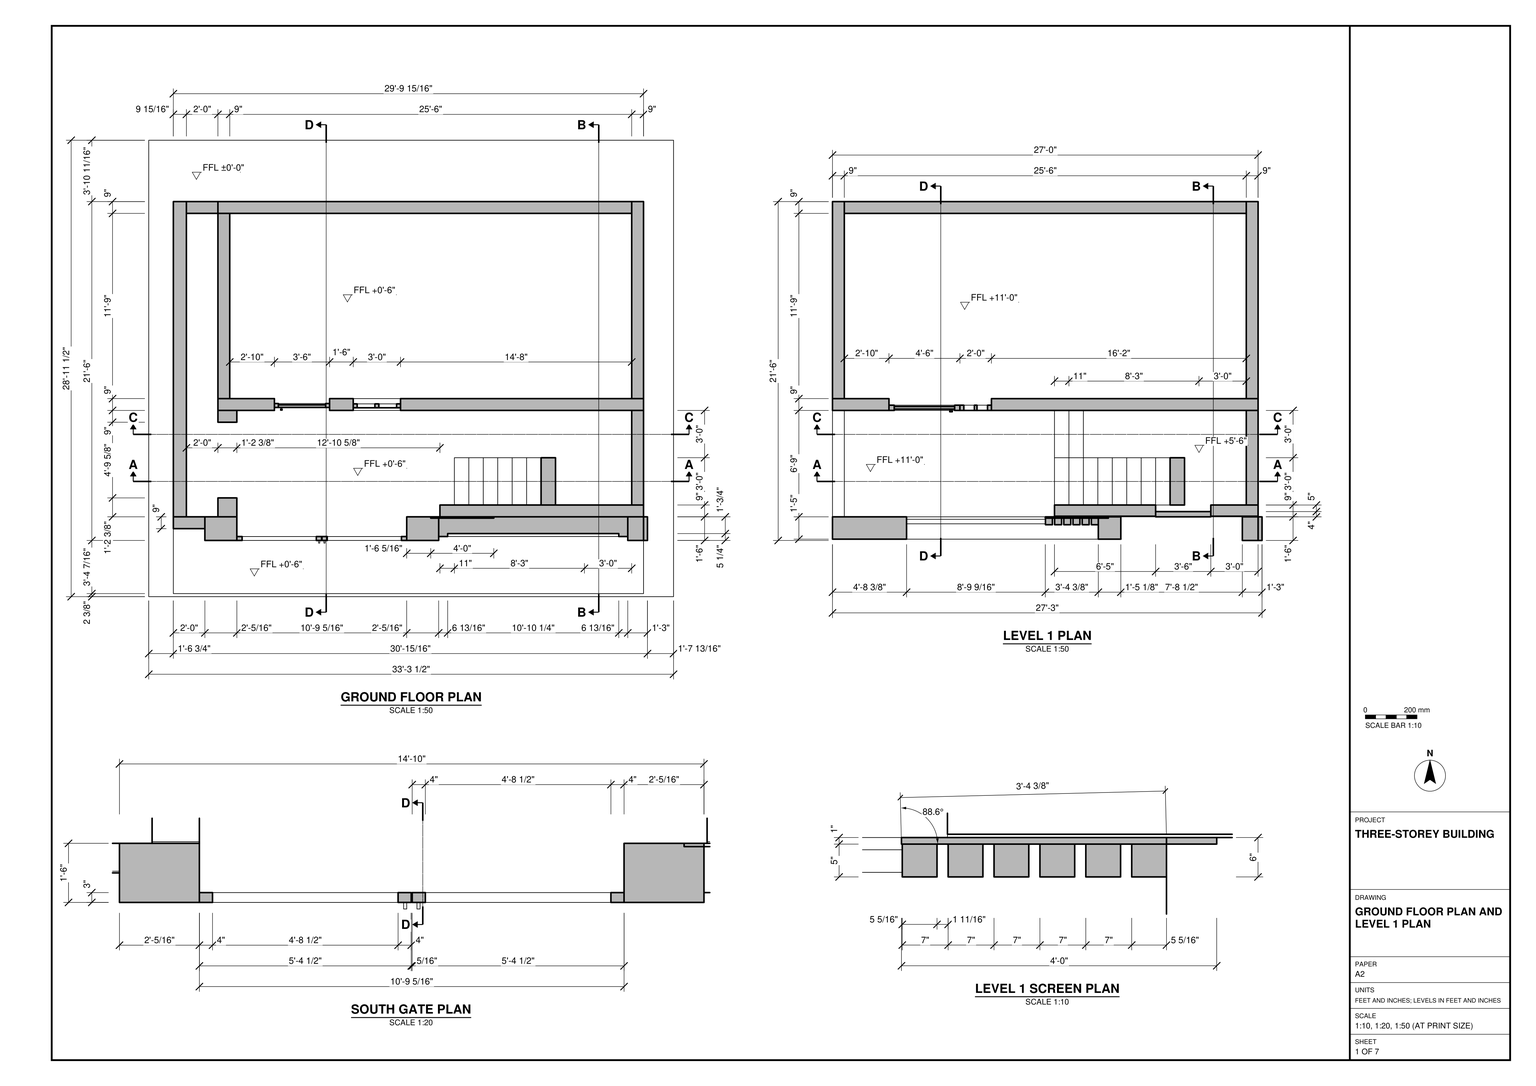
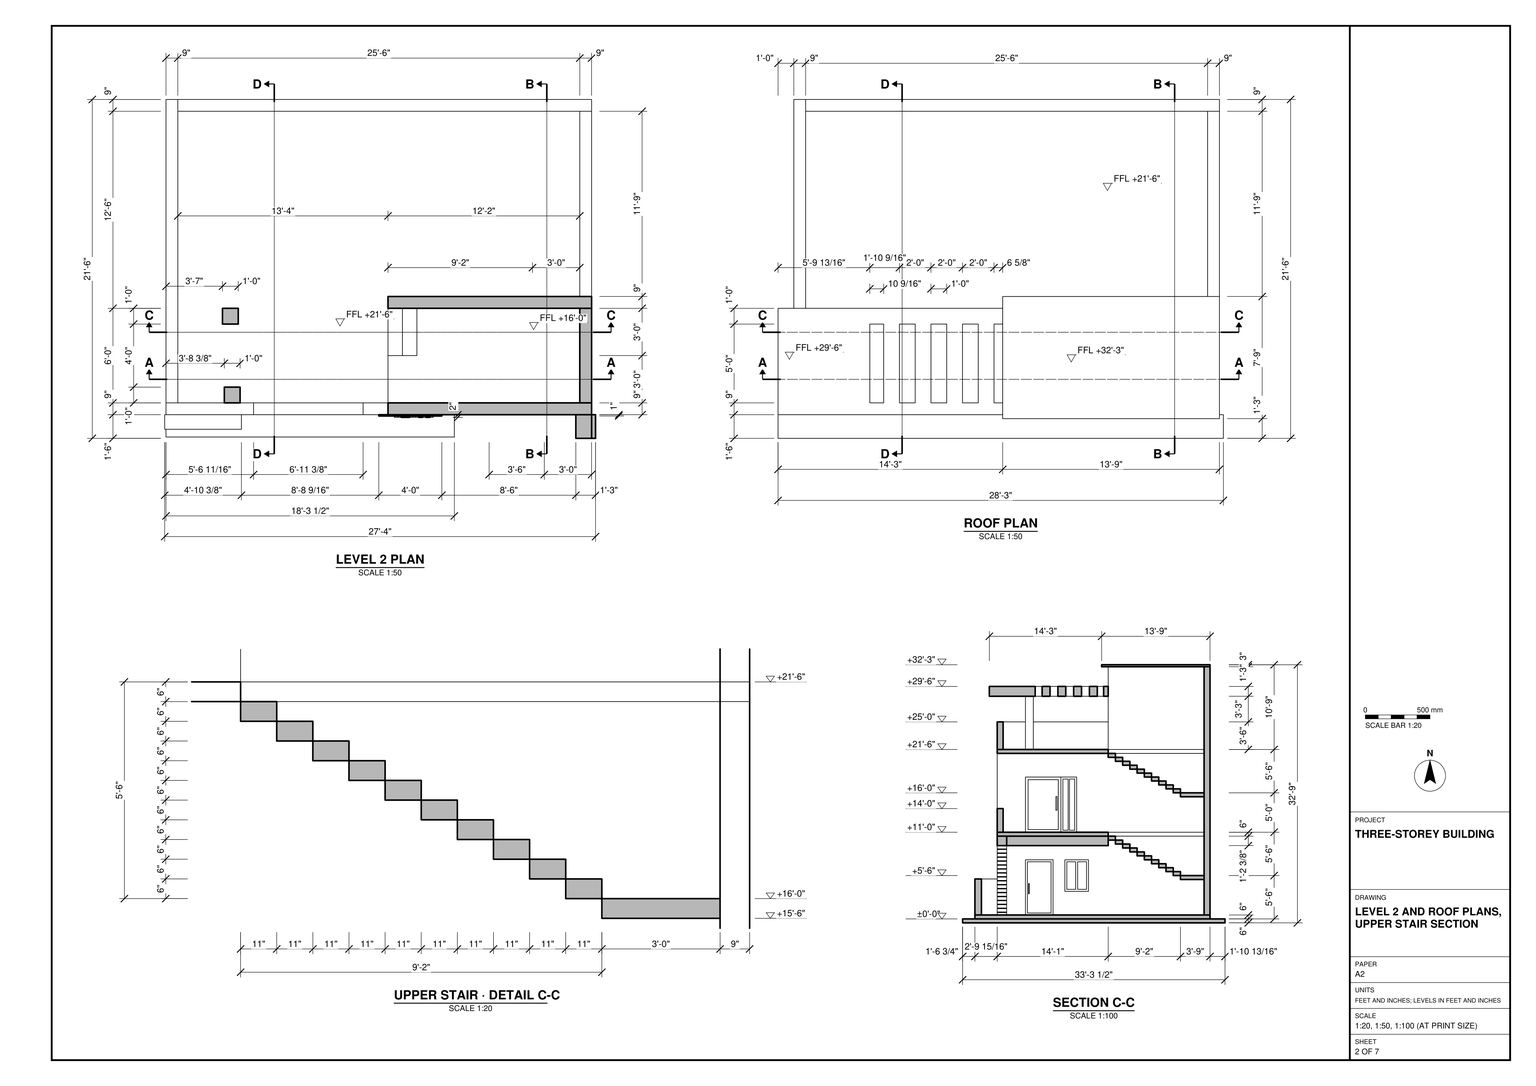
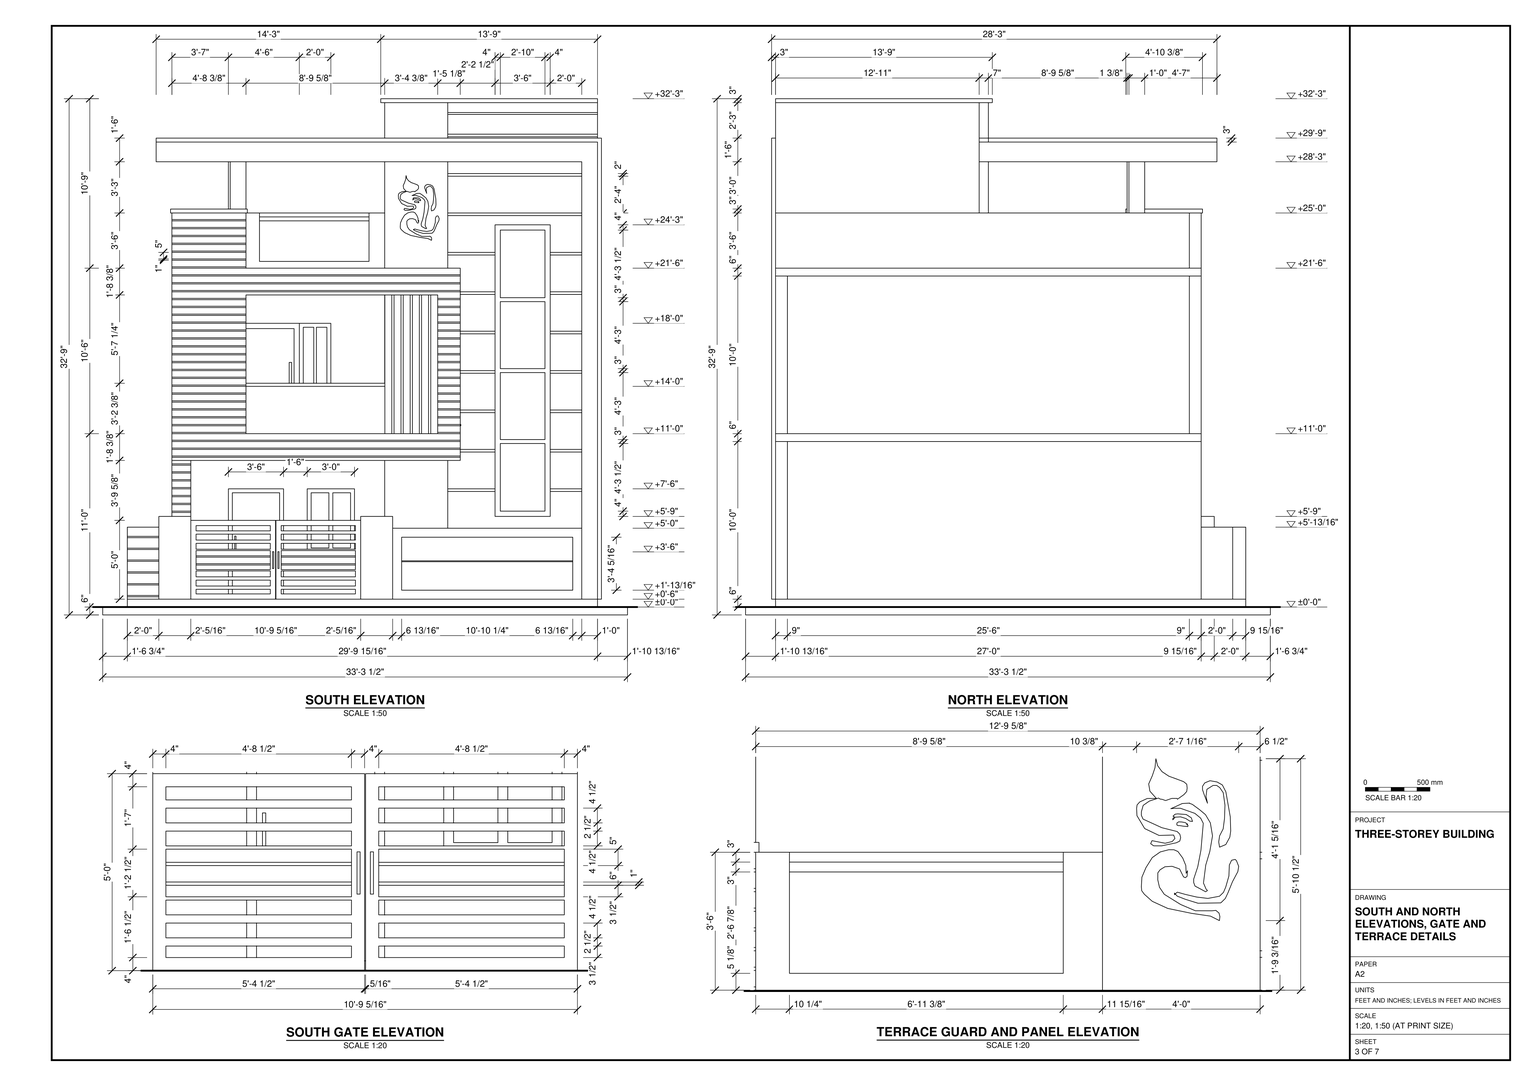
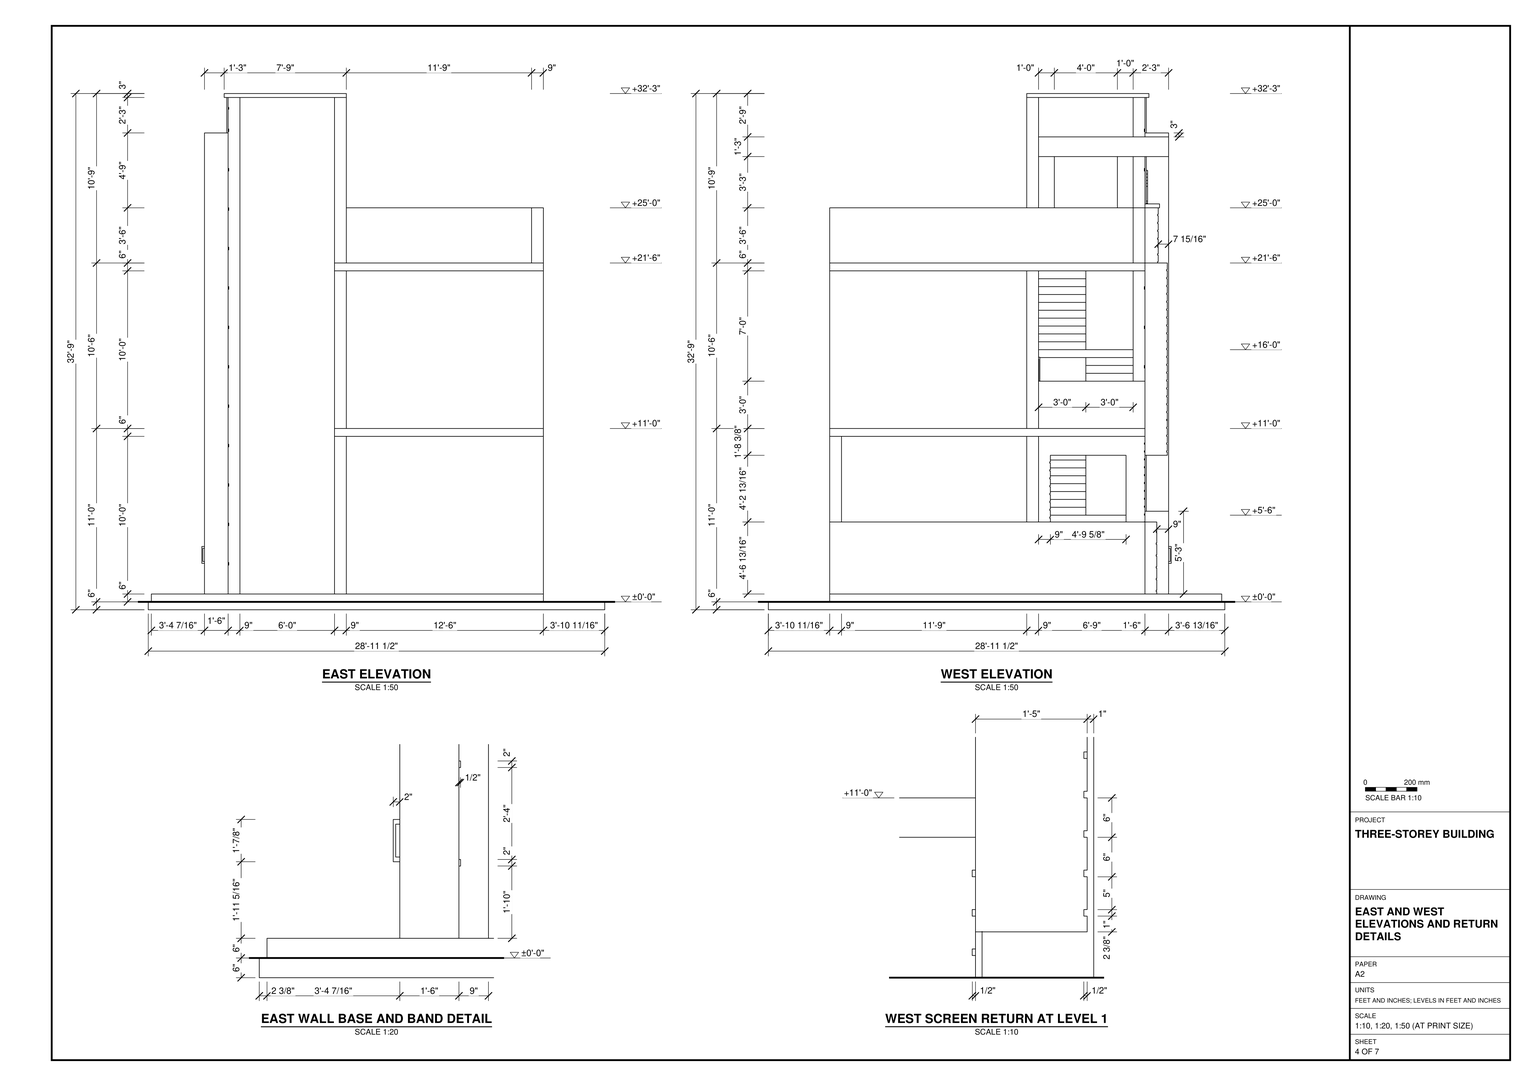
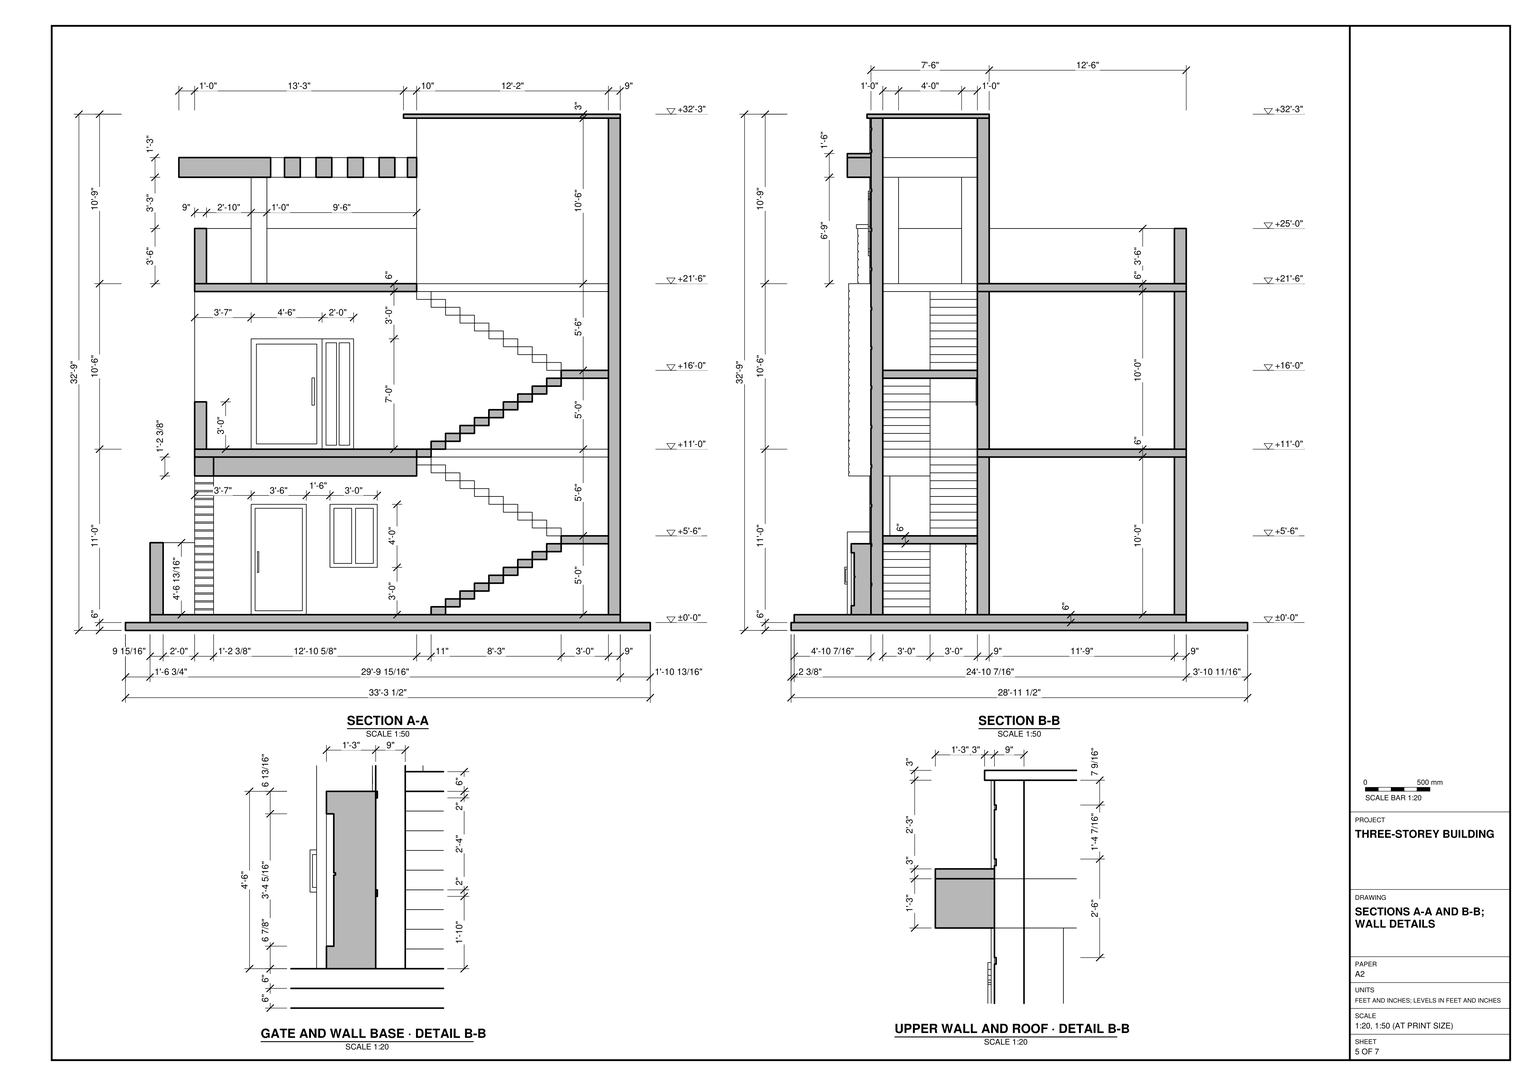
Build the three-storey building in SketchUp from task_files/diagram_01.pdf. Work in feet and inches. Orient the gated frontage to the south. The overall extents, including the base, are 33'-3 1/2" east–west, 28'-11 1/2" north–south and 32'-9" high. Use ±0'-0" as the ground datum, with Level 1 at +11'-0" and Level 2 at +21'-6". Distinguish the raised ground floor at +0'-6" from the surrounding base.

Lay out the walls at the thicknesses shown, with the wide enclosed space to the north and the entrance, stairs and landings to the south. Form the floor slabs around the stair opening and use the sections to connect the flights to their landings. Reproduce the doors and windows in the recessed walls as well as the elements in front of them: the double gate between piers, the horizontally banded balcony frame, the vertical screen and the tall divided panel on the right. At Level 2, model the open terrace, its guard and taller patterned panel. Follow the roof plan for the lower canopy with rectangular openings and the higher solid roof over the stair.

Keep walls, slabs and roof elements in separate groups or components, and group each furniture or joinery piece separately. Use components for repeated parts. Any decor or loose items shown may be suitable library components. Save one SketchUp model as output_files/three_storey_building_with_screened_south_facade.skp.

# SketchUp Ruby script. Lengths in inches.
U = 1.inch
M = Sketchup.active_model
def pt(a) = Geom::Point3d.new(a.map { |v| v * U })
def face(e, loops, mat)
  f = e.add_face(loops[0].map { |a| pt(a) })
  loops[1..].each { |l| e.add_face(l.map { |a| pt(a) }).erase! }
  f.material = f.back_material = mat if mat
  f
end
# faces: each face lists its corners as indices into pts; further lists are holes
def faces(e, pts, list, mat = nil) = list.each { |f| face(e, (f[0].is_a?(Array) ? f : [f]).map { |l| l.map { |i| pts[i] } }, mat) }
# xy, xz, yz: faces in a plane at the given z, y or x. An outline is a flat list of corners, or four numbers for a rectangle; further outlines are holes
def ring(l) = l.size == 4 ? [[l[0], l[1]], [l[2], l[1]], [l[2], l[3]], [l[0], l[3]]] : l.each_slice(2).to_a
def flat(e, list, mat, &to3) = list.each { |f| face(e, (f[0].is_a?(Array) ? f : [f]).map { |l| ring(l).map { |u, v| to3.(u, v) } }, mat) }
def xy(e, z, list, mat = nil) = flat(e, list, mat) { |x, y| [x, y, z] }
def xz(e, y, list, mat = nil) = flat(e, list, mat) { |x, z| [x, y, z] }
def yz(e, x, list, mat = nil) = flat(e, list, mat) { |y, z| [x, y, z] }
def lines(e, pts, list) = list.each { |a, b| e.add_line(pt(pts[a]), pt(pts[b])) }
# prism: a flat outline (further loops are holes) pulled along v
def prism(e, loops, v, mat = nil)
  f = face(e, loops, mat); d = Geom::Vector3d.new(v.map { |x| x * U })
  f.pushpull(f.normal.samedirection?(d) ? d.length : -d.length)
end
def box(e, o, s, mat = nil) = prism(e, [[o, [o[0] + s[0], o[1], o[2]], [o[0] + s[0], o[1] + s[1], o[2]], [o[0], o[1] + s[1], o[2]]]], [0, 0, s[2]], mat)
def at(x, y, z, deg = 0) = Geom::Transformation.translation(pt([x, y, z])) * Geom::Transformation.rotation(ORIGIN, Z_AXIS, deg.degrees)
def axes(o, x, y, z) = Geom::Transformation.new([*x, 0, *y, 0, *z, 0, *pt(o).to_a, 1])
def part(name) = M.definitions.add(name)
# library, detail: a bought-in or finely detailed component or shape, given as its bounding box
def library(name, o, s) = part(name).tap { |d| box(d.entities, o, s) }
def detail(e, o, s) = box(e.add_group.entities, o, s)
def put(e, d, t, mat = nil) = e.add_instance(d, t).tap { |i| i.material = mat if mat }
def group(e, t, mat = nil) = e.add_group.tap { |g| g.transformation = t; g.material = mat if mat }.entities
root = M.entities
M.materials.add("[Color M00]").color = [255, 255, 255]
M.materials.add("[Color M06]").color = [86, 86, 86]
M.materials.add("[Color M07]").color = [58, 58, 58]
M.materials.add("[Metal Silver]").color = [234, 233, 238]
M.materials.add("[Translucent Glass Blue]").color = [100, 149, 237]
M.materials["[Translucent Glass Blue]"].alpha = 0.5
M.materials.add("[Wood Bamboo]").color = [155, 92, 37]
M.materials.add("[Wood Cherry Original]").color = [122, 69, 33]
M.materials.add("[Wood Veneer 01]").color = [86, 50, 26]
c1 = part("Group\#13")
box(c1.entities,[0,0,0],[11,36,6])
c2 = part("Group\#4")
box(c2.entities,[0,0,0],[11,36,6])
c3 = part("Group\#44")
box(c3.entities,[0,0,0],[5.29,5,105.6])
c4 = part("Group\#61")
prism(c4.entities,[[[0.94,2,11.44],[0.94,2,12.875],[0.94,0,12.875],[0.94,0,0],[0.94,2,0],[0.94,2,1.43],[0.94,0.75,1.43],[0.94,0.75,11.44]]],[-0.94,0,0])
c5 = library("Group\#70",[0,0,0],[38.38,2,61.86])
xy(root,44.16,[[100.47,142.05,101.47,144.05]])
xy(root,45.48,[[100.47,142.74,101.47,144.05]])
xy(root,58.65,[[100.47,142.74,101.47,144.05]])
xy(root,60.04,[[100.47,142.05,101.47,144.05]])
xz(root,142.05,[[100.47,44.16,101.47,60.04]],"[Metal Silver]")
xz(root,142.74,[[100.47,45.48,101.47,58.65]])
xz(root,144.05,[[100.47,44.16,101.47,45.48],[100.47,58.65,101.47,60.04]])
yz(root,100.47,[[142.05,44.16,142.05,60.04,144.05,60.04,144.05,58.65,142.74,58.65,142.74,45.48,144.05,45.48,144.05,44.16]])
yz(root,101.47,[[142.05,44.16,144.05,44.16,144.05,45.48,142.74,45.48,142.74,58.65,144.05,58.65,144.05,60.04,142.05,60.04]])
p = [[255.01,60.8,138],[214.66,59.8,138],[214.66,60.8,138],[262.66,60.8,264],[214.66,59.8,264],[262.66,59.8,264],
  [220.71,59.8,75],[214.66,59.8,75],[214.66,60.8,75],[220.71,59.8,66],[262.66,59.8,66],[262.66,60.8,66]]
lines(root,p,[[0,1],[1,2],[3,4],[4,5],[6,7],[7,8],[9,6],[9,10],[10,11]])
g1 = group(root,at(73.125,0,0))
box(g1,[-73.125,0,0],[399.5,347.5,6])
g2 = group(root,at(112.66,60.8,6))
box(g2,[-93.9375,-58.4375,0],[357.9375,298.4375,6])
g3 = group(root,at(232.66,60.8,12))
xy(g3,0,[[-11,0,144,9]])
xy(g3,22,[[-11,0,144,0.5]])
xy(g3,24,[[-11,0,144,0.5]])
xy(g3,52,[[-11,0,144,0.5]])
xy(g3,54,[[-11,0,144,0.5]])
xy(g3,63,[[66,0,108,9]])
xy(g3,82,[[-11,0,66,0.5],[108,0,144,0.5]])
xy(g3,84,[[-11,0,66,0.5],[108,0,144,0.5]])
xy(g3,112,[[-11,0,66,0.5],[108,0,144,0.5]])
xy(g3,114,[[-11,0,66,0.5],[108,0,144,0.5]])
xy(g3,142,[[-11,0,66,0.5],[108,0,144,0.5]])
xy(g3,144,[[-11,0,66,0.5],[108,0,144,0.5]])
xy(g3,172,[[-11,0,66,0.5],[108,0,144,0.5]])
xy(g3,174,[[-11,0,66,0.5],[108,0,144,0.5]])
xy(g3,202,[[-11,0,66,0.5],[108,0,144,0.5]])
xy(g3,204,[[-11,0,66,0.5],[108,0,144,0.5]])
xy(g3,232,[[-11,0,66,0.5],[108,0,144,0.5]])
xy(g3,234,[[-11,0,66,0.5],[108,0,144,0.5]])
xy(g3,262,[[-11,0,66,0.5],[108,0,144,0.5]])
xy(g3,264,[[-11,0,66,0.5],[108,0,144,0.5]])
xy(g3,285,[[66,0,108,9]])
xy(g3,292,[[-11,0,144,0.5]])
xy(g3,294,[[-11,0,144,0.5]])
xy(g3,322,[[-11,0,144,0.5]])
xy(g3,324,[[-11,0,144,0.5]])
xy(g3,352,[[-11,0,144,0.5]])
xy(g3,354,[[-11,0,144,0.5]])
xy(g3,369.03,[[30,0,144,0.5]])
xy(g3,370.46,[[30,0,144,0.5]])
xy(g3,378,[[-11,0,144,9]])
xz(g3,0,[[-11,0,144,22],[-11,24,144,52],[-11,54,144,54,144,82,108,82,108,63,66,63,66,82,-11,82],[-11,84,66,112],[108,84,144,112],
  [-11,114,66,142],[108,114,144,142],[-11,144,66,172],[108,144,144,172],[-11,174,66,202],
  [108,174,144,202],[-11,204,66,232],[108,204,144,232],[-11,234,66,262],[108,234,144,262],
  [-11,264,66,264,66,285,108,285,108,264,144,264,144,292,-11,292],[-11,294,144,322],[-11,324,144,352],[-11,354,144,354,144,369.03,30,369.03,30,370.46,144,370.46,144,378,-11,378]])
xz(g3,0.5,[[-11,22,144,24],[-11,52,144,54],[-11,82,66,84],[108,82,144,84],[-11,112,66,114],
  [108,112,144,114],[-11,142,66,144],[108,142,144,144],[-11,172,66,174],[108,172,144,174],
  [-11,202,66,204],[108,202,144,204],[-11,232,66,234],[108,232,144,234],[-11,262,66,264],
  [108,262,144,264],[-11,292,144,294],[-11,322,144,324],[-11,352,144,354],[30,369.03,144,370.46]])
xz(g3,9,[[[-11,0,144,378],[66,63,108,285]]])
yz(g3,-11,[[0,0,0,22,0.5,22,0.5,24,0,24,0,52,0.5,52,0.5,54,0,54,0,82,0.5,82,0.5,84,0,84,0,112,0.5,112,0.5,114,0,114,0,142,0.5,142,0.5,144,0,144,0,172,0.5,172,0.5,174,0,174,0,202,0.5,202,0.5,204,0,204,0,232,0.5,232,0.5,234,0,234,0,262,0.5,262,0.5,264,0,264,0,292,0.5,292,0.5,294,0,294,0,322,0.5,322,0.5,324,0,324,0,352,0.5,352,0.5,354,0,354,0,378,9,378,9,0]])
yz(g3,30,[[0,369.03,0.5,370.46]])
yz(g3,66,[[0,63,9,63,9,285,0,285,0,264,0.5,264,0.5,262,0,262,0,234,0.5,234,0.5,232,0,232,0,204,0.5,204,0.5,202,0,202,0,174,0.5,174,0.5,172,0,172,0,144,0.5,144,0.5,142,0,142,0,114,0.5,114,0.5,112,0,112,0,84,0.5,84,0.5,82,0,82]])
yz(g3,108,[[0,63,0,82,0.5,82,0.5,84,0,84,0,112,0.5,112,0.5,114,0,114,0,142,0.5,142,0.5,144,0,144,0,172,0.5,172,0.5,174,0,174,0,202,0.5,202,0.5,204,0,204,0,232,0.5,232,0.5,234,0,234,0,262,0.5,262,0.5,264,0,264,0,285,9,285,9,63]])
yz(g3,144,[[0,0,9,0,9,378,0,378,0,370.46,0.5,370.46,0.5,369.03,0,369.03,0,354,0.5,354,0.5,352,0,352,0,324,0.5,324,0.5,322,0,322,0,294,0.5,294,0.5,292,0,292,0,264,0.5,264,0.5,262,0,262,0,234,0.5,234,0.5,232,0,232,0,204,0.5,204,0.5,202,0,202,0,174,0.5,174,0.5,172,0,172,0,144,0.5,144,0.5,142,0,142,0,114,0.5,114,0.5,112,0,112,0,84,0.5,84,0.5,82,0,82,0,54,0.5,54,0.5,52,0,52,0,24,0.5,24,0.5,22,0,22]])
g4 = group(root,at(112.66,141.8,12))
prism(g4,[[[-17,9,0],[-60,9,0],[-60,9,120],[264,9,120],[264,9,0],[25,9,0],[25,9,84],[-17,9,84]],[[79,9,84],[43,9,84],[43,9,36],[79,9,36]]],[0,-9,0])
g5 = group(root,at(367.66,150.8,12))
box(g5,[0,0,0],[9,150,120])
g6 = group(root,at(42.72,291.8,12))
box(g6,[9.9375,0,0],[315,9,120])
g7 = group(root,at(52.66,150.8,12))
box(g7,[0,0,0],[9,141,120])
g8 = group(root,at(52.66,141.8,132))
prism(g8,[[[324,159,0],[324,0,0],[169,0,0],[169,-81,0],[0,-81,0],[0,159,0]]],[0,0,6])
g9 = group(root,at(221.66,69.8,12))
g10 = group(g9,at(11,0,0))
put(g10,c1,at(66,0,36))
put(g10,c1,at(0,0,0))
put(g10,c1,at(55,0,30))
put(g10,c1,at(44,0,24))
put(g10,c1,at(77,0,42))
put(g10,c1,at(88,0,48))
put(g10,c1,at(33,0,18))
put(g10,c1,at(11,0,6))
put(g10,c1,at(22,0,12))
g11 = group(g9,at(110,0,54))
box(g11,[0,0,0],[36,72,6])
put(g9,c1,at(77,72,78,-180))
put(g9,c2,at(11,72,114,-180))
put(g9,c1,at(44,72,96,-180))
put(g9,c1,at(110,72,60,-180))
put(g9,c2,at(22,72,108,-180))
put(g9,c1,at(88,72,72,-180))
put(g9,c1,at(66,72,84,-180))
put(g9,c1,at(99,72,66,-180))
put(g9,c1,at(55,72,90,-180))
put(g9,c1,at(33,72,102,-180))
put(root,c2,at(243.66,141.8,246,-180))
put(root,c1,at(331.66,141.8,198,-180))
put(root,c1,at(309.66,141.8,210,-180))
put(root,c1,at(287.66,141.8,222,-180))
put(root,c1,at(320.66,141.8,204,-180))
put(root,c1,at(276.66,141.8,228,-180))
put(root,c1,at(254.66,141.8,240,-180))
g12 = group(root,at(331.66,69.8,192))
box(g12,[0,0,0],[36,72,6])
put(root,c2,at(232.66,141.8,252,-180))
put(root,c1,at(265.66,141.8,234,-180))
put(root,c1,at(298.66,141.8,216,-180))
put(root,c1,at(298.66,69.8,174))
put(root,c1,at(232.66,69.8,138))
put(root,c1,at(287.66,69.8,168))
put(root,c1,at(309.66,69.8,180))
put(root,c1,at(243.66,69.8,144))
put(root,c1,at(265.66,69.8,156))
put(root,c1,at(254.66,69.8,150))
put(root,c1,at(276.66,69.8,162))
put(root,c1,at(320.66,69.8,186))
put(root,c1,at(221.66,69.8,132))
g13 = group(root,at(52.66,141.8,138))
prism(g13,[[[43,9,0],[0,9,0],[0,9,120],[324,9,120],[324,9,0],[121,9,0],[121,9,84],[43,9,84]]],[0,-9,0])
g14 = group(root,at(367.66,150.8,138))
box(g14,[0,0,0],[9,150,120])
g15 = group(root,at(52.66,150.8,138))
box(g15,[0,0,0],[9,150,120])
g16 = group(root,at(61.66,291.8,138))
box(g16,[0,0,0],[306,9,120])
g17 = group(root,at(52.66,141.8,258))
xy(g17,0,[[0,-81,0,159,324,159,324,0,169,0,169,-81]],"[Wood Cherry Original]")
xy(g17,6,[[0,-81,169,-81,169,0,324,0,324,159,0,159]])
xz(g17,-81,[[0,0,169,6]])
xz(g17,0,[[169,0,324,6]])
xz(g17,159,[[0,0,324,6]])
yz(g17,0,[[-81,0,159,6]])
yz(g17,169,[[-81,0,0,6]])
yz(g17,324,[[0,0,159,6]])
g18 = group(root,at(95.66,144.05,12),"[Color M07]")
prism(g18,[[[0,3,0],[0,3,84],[42,3,84],[42,3,0]],[[39,3,81],[3,3,81],[3,3,3],[39,3,3]]],[0,-3,0])
g19 = group(root,at(98.66,144.05,15),"[Wood Veneer 01]")
box(g19,[0,0,0],[36,2,78])
g20 = group(root,at(155.66,143.8,48),"[Color M07]")
prism(g20,[[[0,0,48],[0,0,0],[36,0,0],[36,0,48]],[[16.5,0,45],[16.5,0,3],[3,0,3],[3,0,45]],[[19.5,0,45],[33,0,45],[33,0,3],[19.5,0,3]]],[0,3,0])
g21 = group(root,at(175.16,143.8,51),"[Translucent Glass Blue]")
xz(g21,0,[[0,0,13.5,42]])
g22 = group(root,at(158.66,143.8,51),"[Translucent Glass Blue]")
xz(g22,0,[[0,0,13.5,42]])
g23 = group(root,at(52.66,60.8,12),"[Wood Bamboo]")
prism(g23,[[[14.4,0.5,0],[14.4,14.4,0],[14.4,14.4,105.6],[14.4,72,105.6],[14.4,72,100.6],[14.4,72.5,100.6],[14.4,72.5,99.6],[14.4,72,99.6],[14.4,72,94.6],[14.4,72.5,94.6],[14.4,72.5,93.6],[14.4,72,93.6],[14.4,72,88.6],[14.4,72.5,88.6],[14.4,72.5,87.6],[14.4,72,87.6],[14.4,72,82.6],[14.4,72.5,82.6],[14.4,72.5,81.6],[14.4,72,81.6],[14.4,72,76.6],[14.4,72.5,76.6],[14.4,72.5,75.6],[14.4,72,75.6],[14.4,72,70.6],[14.4,72.5,70.6],[14.4,72.5,69.6],[14.4,72,69.6],[14.4,72,64.6],[14.4,72.5,64.6],[14.4,72.5,63.6],[14.4,72,63.6],[14.4,72,58.6],[14.4,72.5,58.6],[14.4,72.5,57.6],[14.4,72,57.6],[14.4,72,52.6],[14.4,72.5,52.6],[14.4,72.5,51.6],[14.4,72,51.6],[14.4,72,46.6],[14.4,72.5,46.6],[14.4,72.5,45.6],[14.4,72,45.6],[14.4,72,40.6],[14.4,72.5,40.6],[14.4,72.5,39.6],[14.4,72,39.6],[14.4,72,34.6],[14.4,72.5,34.6],[14.4,72.5,33.6],[14.4,72,33.6],[14.4,72,28.6],[14.4,72.5,28.6],[14.4,72.5,27.6],[14.4,72,27.6],[14.4,72,22.6],[14.4,72.5,22.6],[14.4,72.5,21.6],[14.4,72,21.6],[14.4,72,16.6],[14.4,72.5,16.6],[14.4,72.5,15.6],[14.4,72,15.6],[14.4,72,10.6],[14.4,72.5,10.6],[14.4,72.5,9.6],[14.4,72,9.6],[14.4,72,4.6],[14.4,72.5,4.6],[14.4,72.5,3.6],[14.4,72,3.6],[14.4,72,0],[14.4,81,0],[14.4,81,120],[14.4,0,120],[14.4,0,115],[14.4,0.5,115],[14.4,0.5,114],[14.4,0,114],[14.4,0,109],[14.4,0.5,109],[14.4,0.5,108],[14.4,0,108],[14.4,0,103],[14.4,0.5,103],[14.4,0.5,102],[14.4,0,102],[14.4,0,97],[14.4,0.5,97],[14.4,0.5,96],[14.4,0,96],[14.4,0,91],[14.4,0.5,91],[14.4,0.5,90],[14.4,0,90],[14.4,0,85],[14.4,0.5,85],[14.4,0.5,84],[14.4,0,84],[14.4,0,79],[14.4,0.5,79],[14.4,0.5,78],[14.4,0,78],[14.4,0,73],[14.4,0.5,73],[14.4,0.5,72],[14.4,0,72],[14.4,0,67],[14.4,0.5,67],[14.4,0.5,66],[14.4,0,66],[14.4,0,61],[14.4,0.5,61],[14.4,0.5,60],[14.4,0,60],[14.4,0,55],[14.4,0.5,55],[14.4,0.5,54],[14.4,0,54],[14.4,0,49],[14.4,0.5,49],[14.4,0.5,48],[14.4,0,48],[14.4,0,43],[14.4,0.5,43],[14.4,0.5,42],[14.4,0,42],[14.4,0,37],[14.4,0.5,37],[14.4,0.5,36],[14.4,0,36],[14.4,0,31],[14.4,0.5,31],[14.4,0.5,30],[14.4,0,30],[14.4,0,25],[14.4,0.5,25],[14.4,0.5,24],[14.4,0,24],[14.4,0,19],[14.4,0.5,19],[14.4,0.5,18],[14.4,0,18],[14.4,0,13],[14.4,0.5,13],[14.4,0.5,12],[14.4,0,12],[14.4,0,7],[14.4,0.5,7],[14.4,0.5,6],[14.4,0,6],[14.4,0,1],[14.4,0.5,1]]],[-14.4,0,0])
g24 = group(root,at(67.0625,60.8,117.6))
xy(g24,0,[[0,0,154.6,81]],"[Wood Cherry Original]")
xy(g24,14.4,[[0,0,154.6,81]])
xz(g24,0,[[0,0,154.6,14.4]])
xz(g24,81,[[0,0,154.6,14.4]])
yz(g24,0,[[0,0,81,14.4]])
yz(g24,154.6,[[0,0,81,14.4]])
g25 = group(root,at(298.66,60.8,75),"[Translucent Glass Blue]")
g26 = group(g25,at(4,0,112.5))
xz(g26,0,[[0,0,34,51]])
g27 = group(g25,at(4,0,166.5))
xz(g27,0,[[0,0,34,51.5]])
g28 = group(g25,at(4,0,58.5))
xz(g28,0,[[0,0,34,51]])
g29 = group(g25,at(4,0,4))
xz(g29,0,[[0,0,34,51.5]])
g30 = group(g25,at(0,0,0))
prism(g30,[[[42,4,222],[42,4,0],[0,4,0],[0,4,222]],[[4,4,166.5],[38,4,166.5],[38,4,218],[4,4,218]],[[38,4,4],[38,4,55.5],[4,4,55.5],[4,4,4]],[[38,4,109.5],[4,4,109.5],[4,4,58.5],[38,4,58.5]],[[4,4,163.5],[4,4,112.5],[38,4,112.5],[38,4,163.5]]],[0,-4,0],"[Color M07]")
g31 = group(root,at(367.66,69.8,12))
box(g31,[0,0,0],[9,72,378])
g32 = group(root,at(214.66,59.8,12),"[Color M06]")
box(g32,[0,0,0],[48,1,378])
g33 = group(root,at(364.66,42.8,12))
xy(g33,0,[[0,0,12,18]])
xy(g33,333,[[[-324,0,-324,99,-143,99,-143,18,0,18,0,0],[-231.6,27,-219.6,87],[-207.6,27,-195.6,87],[-183.6,27,-171.6,87],[-254.16,27,-243.6,87],[-159.6,27,-150,87]]])
xy(g33,348,[[[-324,0,12,0,12,18,-143,18,-143,99,-324,99],[-183.6,27,-171.6,87],[-207.6,27,-195.6,87],[-231.6,27,-219.6,87],[-254.16,27,-243.6,87],[-159.6,27,-150,87]]])
xz(g33,0,[[0,0,12,0,12,348,-324,348,-324,333,0,333]])
xz(g33,18,[[0,0,0,333,-143,333,-143,348,12,348,12,0]])
xz(g33,27,[[-254.16,333,-243.6,348],[-231.6,333,-219.6,348],[-207.6,333,-195.6,348],[-183.6,333,-171.6,348],[-159.6,333,-150,348]])
xz(g33,87,[[-254.16,333,-243.6,348],[-231.6,333,-219.6,348],[-207.6,333,-195.6,348],[-183.6,333,-171.6,348],[-159.6,333,-150,348]])
xz(g33,99,[[-324,333,-143,348]])
yz(g33,-324,[[0,333,99,348]])
yz(g33,-254.16,[[27,333,87,348]])
yz(g33,-243.6,[[27,333,87,348]])
yz(g33,-231.6,[[27,333,87,348]])
yz(g33,-219.6,[[27,333,87,348]])
yz(g33,-207.6,[[27,333,87,348]])
yz(g33,-195.6,[[27,333,87,348]])
yz(g33,-183.6,[[27,333,87,348]])
yz(g33,-171.6,[[27,333,87,348]])
yz(g33,-159.6,[[27,333,87,348]])
yz(g33,-150,[[27,333,87,348]])
yz(g33,-143,[[18,333,99,348]])
yz(g33,0,[[0,0,18,333]])
yz(g33,12,[[0,0,18,348]])
g34 = group(root,at(376.66,42.8,12),"[Color M06]")
prism(g34,[[[0,18,0],[0,18,348],[-336,18,348],[-336,18,351],[3,18,351],[3,18,0]]],[0,-18,0])
g35 = group(root,at(95.66,141.8,138),"[Color M07]")
prism(g35,[[[0,4,0],[0,4,84],[54,4,84],[54,4,0]],[[50,4,4],[50,4,80],[4,4,80],[4,4,4]]],[0,-4,0])
g36 = group(root,at(149.66,141.8,138),"[Color M07]")
prism(g36,[[[0,4,84],[24,4,84],[24,4,0],[0,4,0]],[[11,4,3],[11,4,81],[3,4,81],[3,4,3]],[[21,4,81],[13,4,81],[13,4,3],[21,4,3]]],[0,-4,0])
g37 = group(root,at(162.66,141.8,141),"[Translucent Glass Blue]")
xz(g37,0,[[0,0,8,78]])
g38 = group(root,at(152.66,141.8,141),"[Translucent Glass Blue]")
xz(g38,0,[[0,0,8,78]])
g39 = group(root,at(99.66,142.8,142),"[Wood Veneer 01]")
box(g39,[0,0,0],[46,2,76])
g40 = group(root,at(141.95,140.8,171.49),"[Metal Silver]")
prism(g40,[[[1.875,2,19.25],[1.875,2,20.75],[1.875,0,20.75],[1.875,0,0],[1.875,2,0],[1.875,2,1.5],[1.875,0.75,1.5],[1.875,0.75,19.25]]],[-1.875,0,0])
g41 = group(root,at(52.66,48.8,117.6),"[Wood Bamboo]")
xy(g41,0,[[0,-5,219.5,12]])
xy(g41,2.4,[[0,-5,219.5,-4.5]])
xy(g41,3.4,[[0,-5,219.5,-4.5]])
xy(g41,8.4,[[0,-5,219.5,-4.5]])
xy(g41,9.4,[[0,-5,219.5,-4.5]])
xy(g41,14.4,[[0,-5,219.5,-4.5]])
xy(g41,15.4,[[0,-5,219.5,-4.5]])
xy(g41,20.4,[[0,-5,56.4,-4.5],[56.4,-5,202.35,12],[202.35,-5,219.5,-4.5]])
xy(g41,21.4,[[0,-5,56.4,-4.5],[202.35,-5,219.5,-4.5]])
xy(g41,26.4,[[0,-5,56.4,-4.5],[202.35,-5,219.5,-4.5]])
xy(g41,27.4,[[0,-5,56.4,-4.5],[202.35,-5,219.5,-4.5]])
xy(g41,32.4,[[0,-5,56.4,-4.5],[202.35,-5,219.5,-4.5]])
xy(g41,33.4,[[0,-5,56.4,-4.5],[202.35,-5,219.5,-4.5]])
xy(g41,38.4,[[0,-5,56.4,-4.5],[202.35,-5,219.5,-4.5]])
xy(g41,39.4,[[0,-5,56.4,-4.5],[202.35,-5,219.5,-4.5]])
xy(g41,44.4,[[0,-5,56.4,-4.5],[202.35,-5,219.5,-4.5]])
xy(g41,45.4,[[0,-5,56.4,-4.5],[202.35,-5,219.5,-4.5]])
xy(g41,50.4,[[0,-5,56.4,-4.5],[202.35,-5,219.5,-4.5]])
xy(g41,51.4,[[0,-5,56.4,-4.5],[202.35,-5,219.5,-4.5]])
xy(g41,56.4,[[0,-5,56.4,-4.5],[202.35,-5,219.5,-4.5]])
xy(g41,57.4,[[0,-5,56.4,-4.5],[202.35,-5,219.5,-4.5]])
xy(g41,62.4,[[0,-5,56.4,-4.5],[202.35,-5,219.5,-4.5]])
xy(g41,63.4,[[0,-5,56.4,-4.5],[202.35,-5,219.5,-4.5]])
xy(g41,68.4,[[0,-5,56.4,-4.5],[202.35,-5,219.5,-4.5]])
xy(g41,69.4,[[0,-5,56.4,-4.5],[202.35,-5,219.5,-4.5]])
xy(g41,74.4,[[0,-5,56.4,-4.5],[202.35,-5,219.5,-4.5]])
xy(g41,75.4,[[0,-5,56.4,-4.5],[202.35,-5,219.5,-4.5]])
xy(g41,80.4,[[0,-5,56.4,-4.5],[202.35,-5,219.5,-4.5]])
xy(g41,81.4,[[0,-5,56.4,-4.5],[202.35,-5,219.5,-4.5]])
xy(g41,86.4,[[0,-5,56.4,-4.5],[202.35,-5,219.5,-4.5]])
xy(g41,87.4,[[0,-5,56.4,-4.5],[202.35,-5,219.5,-4.5]])
xy(g41,92.4,[[0,-5,56.4,-4.5],[202.35,-5,219.5,-4.5]])
xy(g41,93.4,[[0,-5,56.4,-4.5],[202.35,-5,219.5,-4.5]])
xy(g41,98.4,[[0,-5,56.4,-4.5],[202.35,-5,219.5,-4.5]])
xy(g41,99.4,[[0,-5,56.4,-4.5],[202.35,-5,219.5,-4.5]])
xy(g41,104.4,[[0,-5,56.4,-4.5],[202.35,-5,219.5,-4.5]])
xy(g41,105.4,[[0,-5,56.4,-4.5],[202.35,-5,219.5,-4.5]])
xy(g41,110.4,[[0,-5,56.4,-4.5],[202.35,-5,219.5,-4.5]])
xy(g41,111.4,[[0,-5,56.4,-4.5],[202.35,-5,219.5,-4.5]])
xy(g41,116.4,[[0,-5,56.4,-4.5],[202.35,-5,219.5,-4.5]])
xy(g41,117.4,[[0,-5,56.4,-4.5],[202.35,-5,219.5,-4.5]])
xy(g41,122.4,[[0,-5,56.4,-4.5],[202.35,-5,219.5,-4.5]])
xy(g41,123.4,[[0,-5,56.4,-4.5],[202.35,-5,219.5,-4.5]])
xy(g41,126,[[56.4,-5,202.35,12]])
xy(g41,128.4,[[0,-5,219.5,-4.5]])
xy(g41,129.4,[[0,-5,219.5,-4.5]])
xy(g41,134.4,[[0,-5,219.5,-4.5]])
xy(g41,135.4,[[0,-5,219.5,-4.5]])
xy(g41,140.4,[[0,-5,219.5,-4.5]])
xy(g41,141.4,[[0,-5,219.5,-4.5]])
xy(g41,146.4,[[0,-5,219.5,12]])
xz(g41,-5,[[0,0,219.5,2.4],[0,3.4,219.5,8.4],[0,9.4,219.5,14.4],[0,15.4,219.5,20.4],[0,21.4,56.4,26.4],
  [202.35,21.4,219.5,26.4],[219.5,26.4,219.96,27.4],[0,27.4,56.4,32.4],[202.35,27.4,219.5,32.4],[0,33.4,56.4,38.4],
  [202.35,33.4,219.5,38.4],[0,39.4,56.4,44.4],[202.35,39.4,219.5,44.4],[0,45.4,56.4,50.4],[202.35,45.4,219.5,50.4],
  [0,51.4,56.4,56.4],[202.35,51.4,219.5,56.4],[0,57.4,56.4,62.4],[202.35,57.4,219.5,62.4],[0,63.4,56.4,68.4],
  [202.35,63.4,219.5,68.4],[0,69.4,56.4,74.4],[202.35,69.4,219.5,74.4],[0,75.4,56.4,80.4],[202.35,75.4,219.5,80.4],
  [0,81.4,56.4,86.4],[202.35,81.4,219.5,86.4],[0,87.4,56.4,92.4],[202.35,87.4,219.5,92.4],[0,93.4,56.4,98.4],
  [202.35,93.4,219.5,98.4],[0,99.4,56.4,104.4],[202.35,99.4,219.5,104.4],[0,105.4,56.4,110.4],[202.35,105.4,219.5,110.4],
  [0,111.4,56.4,116.4],[202.35,111.4,219.5,116.4],[0,117.4,56.4,122.4],[202.35,117.4,219.5,122.4],[0,123.4,56.4,123.4,56.4,126,202.35,126,202.35,123.4,219.5,123.4,219.5,128.4,0,128.4],
  [0,129.4,219.5,134.4],[0,135.4,219.5,140.4],[0,141.4,219.5,146.4]])
xz(g41,-4.5,[[0,2.4,219.5,3.4],[0,8.4,219.5,9.4],[0,14.4,219.5,15.4],[0,20.4,56.4,21.4],[202.35,20.4,219.5,21.4],
  [0,26.4,56.4,27.4],[202.35,26.4,219.5,27.4],[0,32.4,56.4,33.4],[202.35,32.4,219.5,33.4],[0,38.4,56.4,39.4],
  [202.35,38.4,219.5,39.4],[0,44.4,56.4,45.4],[202.35,44.4,219.5,45.4],[0,50.4,56.4,51.4],[202.35,50.4,219.5,51.4],
  [0,56.4,56.4,57.4],[202.35,56.4,219.5,57.4],[0,62.4,56.4,63.4],[202.35,62.4,219.5,63.4],[0,68.4,56.4,69.4],
  [202.35,68.4,219.5,69.4],[0,74.4,56.4,75.4],[202.35,74.4,219.5,75.4],[0,80.4,56.4,81.4],[202.35,80.4,219.5,81.4],
  [0,86.4,56.4,87.4],[202.35,86.4,219.5,87.4],[0,92.4,56.4,93.4],[202.35,92.4,219.5,93.4],[0,98.4,56.4,99.4],
  [202.35,98.4,219.5,99.4],[0,104.4,56.4,105.4],[202.35,104.4,219.5,105.4],[0,110.4,56.4,111.4],[202.35,110.4,219.5,111.4],
  [0,116.4,56.4,117.4],[202.35,116.4,219.5,117.4],[0,122.4,56.4,123.4],[202.35,122.4,219.5,123.4],[0,128.4,219.5,129.4],
  [0,134.4,219.5,135.4],[0,140.4,219.5,141.4]])
xz(g41,12,[[[0,0,219.5,146.4],[56.4,20.4,202.35,126]]])
yz(g41,0,[[-5,0,-5,2.4,-4.5,2.4,-4.5,3.4,-5,3.4,-5,8.4,-4.5,8.4,-4.5,9.4,-5,9.4,-5,14.4,-4.5,14.4,-4.5,15.4,-5,15.4,-5,20.4,-4.5,20.4,-4.5,21.4,-5,21.4,-5,26.4,-4.5,26.4,-4.5,27.4,-5,27.4,-5,32.4,-4.5,32.4,-4.5,33.4,-5,33.4,-5,38.4,-4.5,38.4,-4.5,39.4,-5,39.4,-5,44.4,-4.5,44.4,-4.5,45.4,-5,45.4,-5,50.4,-4.5,50.4,-4.5,51.4,-5,51.4,-5,56.4,-4.5,56.4,-4.5,57.4,-5,57.4,-5,62.4,-4.5,62.4,-4.5,63.4,-5,63.4,-5,68.4,-4.5,68.4,-4.5,69.4,-5,69.4,-5,74.4,-4.5,74.4,-4.5,75.4,-5,75.4,-5,80.4,-4.5,80.4,-4.5,81.4,-5,81.4,-5,86.4,-4.5,86.4,-4.5,87.4,-5,87.4,-5,92.4,-4.5,92.4,-4.5,93.4,-5,93.4,-5,98.4,-4.5,98.4,-4.5,99.4,-5,99.4,-5,104.4,-4.5,104.4,-4.5,105.4,-5,105.4,-5,110.4,-4.5,110.4,-4.5,111.4,-5,111.4,-5,116.4,-4.5,116.4,-4.5,117.4,-5,117.4,-5,122.4,-4.5,122.4,-4.5,123.4,-5,123.4,-5,128.4,-4.5,128.4,-4.5,129.4,-5,129.4,-5,134.4,-4.5,134.4,-4.5,135.4,-5,135.4,-5,140.4,-4.5,140.4,-4.5,141.4,-5,141.4,-5,146.4,12,146.4,12,0]])
yz(g41,56.4,[[-4.5,20.4,12,20.4,12,126,-5,126,-5,123.4,-4.5,123.4,-4.5,122.4,-5,122.4,-5,117.4,-4.5,117.4,-4.5,116.4,-5,116.4,-5,111.4,-4.5,111.4,-4.5,110.4,-5,110.4,-5,105.4,-4.5,105.4,-4.5,104.4,-5,104.4,-5,99.4,-4.5,99.4,-4.5,98.4,-5,98.4,-5,93.4,-4.5,93.4,-4.5,92.4,-5,92.4,-5,87.4,-4.5,87.4,-4.5,86.4,-5,86.4,-5,81.4,-4.5,81.4,-4.5,80.4,-5,80.4,-5,75.4,-4.5,75.4,-4.5,74.4,-5,74.4,-5,69.4,-4.5,69.4,-4.5,68.4,-5,68.4,-5,63.4,-4.5,63.4,-4.5,62.4,-5,62.4,-5,57.4,-4.5,57.4,-4.5,56.4,-5,56.4,-5,51.4,-4.5,51.4,-4.5,50.4,-5,50.4,-5,45.4,-4.5,45.4,-4.5,44.4,-5,44.4,-5,39.4,-4.5,39.4,-4.5,38.4,-5,38.4,-5,33.4,-4.5,33.4,-4.5,32.4,-5,32.4,-5,27.4,-4.5,27.4,-4.5,26.4,-5,26.4,-5,21.4,-4.5,21.4]])
yz(g41,202.35,[[-4.5,20.4,-4.5,21.4,-5,21.4,-5,26.4,-4.5,26.4,-4.5,27.4,-5,27.4,-5,32.4,-4.5,32.4,-4.5,33.4,-5,33.4,-5,38.4,-4.5,38.4,-4.5,39.4,-5,39.4,-5,44.4,-4.5,44.4,-4.5,45.4,-5,45.4,-5,50.4,-4.5,50.4,-4.5,51.4,-5,51.4,-5,56.4,-4.5,56.4,-4.5,57.4,-5,57.4,-5,62.4,-4.5,62.4,-4.5,63.4,-5,63.4,-5,68.4,-4.5,68.4,-4.5,69.4,-5,69.4,-5,74.4,-4.5,74.4,-4.5,75.4,-5,75.4,-5,80.4,-4.5,80.4,-4.5,81.4,-5,81.4,-5,86.4,-4.5,86.4,-4.5,87.4,-5,87.4,-5,92.4,-4.5,92.4,-4.5,93.4,-5,93.4,-5,98.4,-4.5,98.4,-4.5,99.4,-5,99.4,-5,104.4,-4.5,104.4,-4.5,105.4,-5,105.4,-5,110.4,-4.5,110.4,-4.5,111.4,-5,111.4,-5,116.4,-4.5,116.4,-4.5,117.4,-5,117.4,-5,122.4,-4.5,122.4,-4.5,123.4,-5,123.4,-5,126,12,126,12,20.4]])
yz(g41,219.5,[[-5,0,12,0,12,146.4,-5,146.4,-5,141.4,-4.5,141.4,-4.5,140.4,-5,140.4,-5,135.4,-4.5,135.4,-4.5,134.4,-5,134.4,-5,129.4,-4.5,129.4,-4.5,128.4,-5,128.4,-5,123.4,-4.5,123.4,-4.5,122.4,-5,122.4,-5,117.4,-4.5,117.4,-4.5,116.4,-5,116.4,-5,111.4,-4.5,111.4,-4.5,110.4,-5,110.4,-5,105.4,-4.5,105.4,-4.5,104.4,-5,104.4,-5,99.4,-4.5,99.4,-4.5,98.4,-5,98.4,-5,93.4,-4.5,93.4,-4.5,92.4,-5,92.4,-5,87.4,-4.5,87.4,-4.5,86.4,-5,86.4,-5,81.4,-4.5,81.4,-4.5,80.4,-5,80.4,-5,75.4,-4.5,75.4,-4.5,74.4,-5,74.4,-5,69.4,-4.5,69.4,-4.5,68.4,-5,68.4,-5,63.4,-4.5,63.4,-4.5,62.4,-5,62.4,-5,57.4,-4.5,57.4,-4.5,56.4,-5,56.4,-5,51.4,-4.5,51.4,-4.5,50.4,-5,50.4,-5,45.4,-4.5,45.4,-4.5,44.4,-5,44.4,-5,39.4,-4.5,39.4,-4.5,38.4,-5,38.4,-5,33.4,-4.5,33.4,-4.5,32.4,-5,32.4,-5,27.4,-4.5,27.4,-4.5,26.4,-5,26.4,-5,21.4,-4.5,21.4,-4.5,20.4,-5,20.4,-5,15.4,-4.5,15.4,-4.5,14.4,-5,14.4,-5,9.4,-4.5,9.4,-4.5,8.4,-5,8.4,-5,3.4,-4.5,3.4,-4.5,2.4,-5,2.4],[-5,26.4,-4.5,27.4]])
put(root,c3,at(249.72,54.8,138),"[Wood Bamboo]")
put(root,c3,at(242.73,54.8,138),"[Wood Bamboo]")
put(root,c3,at(235.74,54.8,138),"[Wood Bamboo]")
put(root,c3,at(228.76,54.8,138),"[Wood Bamboo]")
put(root,c3,at(221.77,54.8,138),"[Wood Bamboo]")
put(root,c3,at(214.78,54.8,138),"[Wood Bamboo]")
g42 = group(root,at(109.0625,57.3,138),"[Translucent Glass Blue]")
xz(g42,0,[[0,0,105.72,36]])
g43 = group(root,at(109.0625,55.5,174),"[Color M06]")
box(g43,[0,0,0],[105.72,3.4375,2.375])
g44 = group(root,at(52.66,60.8,264))
prism(g44,[[[169,9,0],[0,9,0],[0,9,42],[66.68,9,42],[66.68,9,5.125],[150.05,9,5.125],[150.05,9,42],[169,9,42]]],[0,-9,0])
g45 = group(root,at(52.66,50.71,264),"[Wood Bamboo]")
prism(g45,[[[56.4,0.5,0],[56.4,10.09,0],[56.4,10.09,42],[56.4,0,42],[56.4,0,37],[56.4,0.5,37],[56.4,0.5,36],[56.4,0,36],[56.4,0,31],[56.4,0.5,31],[56.4,0.5,30],[56.4,0,30],[56.4,0,25],[56.4,0.5,25],[56.4,0.5,24],[56.4,0,24],[56.4,0,19],[56.4,0.5,19],[56.4,0.5,18],[56.4,0,18],[56.4,0,13],[56.4,0.5,13],[56.4,0.5,12],[56.4,0,12],[56.4,0,7],[56.4,0.5,7],[56.4,0.5,6],[56.4,0,6],[56.4,0,1],[56.4,0.5,1]]],[-56.4,0,0])
g46 = group(root,at(119.34,65.3,269.125),"[Translucent Glass Blue]")
xz(g46,0,[[0,0,83.375,30.875]])
g47 = group(root,at(119.34,60.8,300),"[Color M06]")
box(g47,[0,0,0],[83.375,9,3])
g48 = group(root,at(97.0625,69.8,264))
box(g48,[0,0,0],[12,12,81])
g49 = group(root,at(95.66,129.8,264))
box(g49,[0,0,0],[12,12,81])
g50 = group(root,at(221.66,60.8,264),"[Color M06]")
xy(g50,0,[[0,81,155,90]])
xy(g50,126,[[-10,-3,-10,90,0,90,0,81,155,81,155,-3],[0,81,155,90]])
xy(g50,129,[[-10,-3,155,90]])
xz(g50,-3,[[-10,126,155,129]])
xz(g50,81,[[0,0,155,126]],"[Color M00]")
xz(g50,90,[[-10,126,155,129]])
xz(g50,90,[[0,0,155,126]],"[Color M00]")
yz(g50,-10,[[-3,126,90,129]])
yz(g50,0,[[81,0,90,126]],"[Color M00]")
yz(g50,155,[[-3,126,90,129]])
yz(g50,155,[[81,0,90,126]],"[Color M00]")
g51 = group(root,at(51.66,49.71,306),"[Color M06]")
box(g51,[0,0,0],[58.4,11.09,3])
g52 = group(root,at(42.72,42.8,12),"[Color M06]")
box(g52,[0,0,0],[24.34,18,63])
g53 = group(root,at(196.375,42.8,12),"[Color M06]")
box(g53,[0,0,0],[24.34,18,63])
g54 = group(root,at(220.71,42.8,12))
xy(g54,0,[[0,3,143.95,18]])
xy(g54,6.84,[[6.84,3,137.11,5.25]])
xy(g54,28.51,[[6.84,5.25,137.11,5.75]])
xy(g54,29.2,[[6.84,5.25,137.11,5.75]])
xy(g54,47.16,[[6.84,3,137.11,5.25]])
xy(g54,54,[[0,3,143.95,18]],"[Color M06]")
xz(g54,3,[[[0,0,143.95,54],[6.84,6.84,137.11,47.16]]],"[Color M06]")
xz(g54,5.25,[[6.84,6.84,137.11,28.51],[6.84,29.2,137.11,47.16]])
xz(g54,5.75,[[6.84,28.51,137.11,29.2]])
xz(g54,18,[[0,0,143.95,54]])
yz(g54,0,[[3,0,3,54,17.1,54,18,0],[18,0,17.1,54,18,54]])
yz(g54,6.84,[[3,6.84,5.25,6.84,5.25,28.51,5.75,28.51,5.75,29.2,5.25,29.2,5.25,47.16,3,47.16]])
yz(g54,137.11,[[3,6.84,3,47.16,5.25,47.16,5.25,29.2,5.75,29.2,5.75,28.51,5.25,28.51,5.25,6.84]])
yz(g54,143.95,[[3,0,18,54]])
p = [[0,17.1,54],[0,17,60]]
lines(g54,p,[[0,1]])
g55 = group(root,at(67.0625,42.8,12),"[Color M06]")
prism(g55,[[[0,3,60],[64.51,3,60],[64.51,3,0],[0,3,0]],[[4,3,22.5],[60.51,3,22.5],[60.51,3,37],[4,3,37]],[[4,3,45],[60.51,3,45],[60.51,3,49.5],[4,3,49.5]],[[4,3,38],[60.51,3,38],[60.51,3,42.5],[4,3,42.5]],[[4,3,17],[60.51,3,17],[60.51,3,21.5],[4,3,21.5]],[[4,3,10],[60.51,3,10],[60.51,3,14.5],[4,3,14.5]],[[4,3,52],[60.51,3,52],[60.51,3,56],[4,3,56]],[[60.51,3,4],[60.51,3,7.5],[4,3,7.5],[4,3,4]]],[0,-3,0])
g56 = group(root,at(131.87,42.8,12),"[Color M06]")
prism(g56,[[[0,0,0],[64.51,0,0],[64.51,0,60],[0,0,60]],[[60.51,0,22.5],[4,0,22.5],[4,0,37],[60.51,0,37]],[[60.51,0,45],[4,0,45],[4,0,49.5],[60.51,0,49.5]],[[4,0,38],[4,0,42.5],[60.51,0,42.5],[60.51,0,38]],[[60.51,0,10],[4,0,10],[4,0,14.5],[60.51,0,14.5]],[[4,0,17],[4,0,21.5],[60.51,0,21.5],[60.51,0,17]],[[60.51,0,52],[4,0,52],[4,0,56],[60.51,0,56]],[[60.51,0,7.5],[60.51,0,4],[4,0,4],[4,0,7.5]]],[0,3,0])
g57 = group(root,at(71.0625,42.8,34.5),"[Wood Bamboo]")
prism(g57,[[[56.51,3,0],[56.51,3,14.5],[56.51,0,14.5],[56.51,0,10.5],[56.51,0.5,10.5],[56.51,0.5,9.5],[56.51,0,9.5],[56.51,0,4.5],[56.51,0.5,4.5],[56.51,0.5,3.5],[56.51,0,3.5],[56.51,0,0]]],[-56.51,0,0])
g58 = group(root,at(135.87,42.8,34.5),"[Wood Bamboo]")
prism(g58,[[[56.51,3,0],[56.51,3,14.5],[56.51,0,14.5],[56.51,0,10.5],[56.51,0.5,10.5],[56.51,0.5,9.5],[56.51,0,9.5],[56.51,0,4.5],[56.51,0.5,4.5],[56.51,0.5,3.5],[56.51,0,3.5],[56.51,0,0]]],[-56.51,0,0])
put(root,c4,at(129.26,40.8,35.3125),"[Metal Silver]")
put(root,c4,at(133.32,40.8,35.3125),"[Metal Silver]")
g59 = group(root,at(18.72,60.8,12))
box(g59,[0,0,0],[9.9375,240,54.8125])
g60 = group(root,at(18.72,51.8,12))
prism(g60,[[[24,0,0],[24,9,0],[24,9,54.8125],[24,0,54.8125],[24,0,47.8125],[24,0.5,47.8125],[24,0.5,46.8125],[24,0,46.8125],[24,0,38.8125],[24,0.5,38.8125],[24,0.5,37.8125],[24,0,37.8125],[24,0,29.8125],[24,0.5,29.8125],[24,0.5,28.8125],[24,0,28.8125],[24,0,20.8125],[24,0.5,20.8125],[24,0.5,19.8125],[24,0,19.8125],[24,0,11.8125],[24,0.5,11.8125],[24,0.5,10.8125],[24,0,10.8125],[24,0,2.8125],[24,0.5,2.8125],[24,0.5,1.8125],[24,0,1.8125]]],[-24,0,0])
g61 = group(root,at(28.66,291.8,12))
box(g61,[0,0,0],[24,9,54.8125])
g62 = group(root,at(52.66,60.8,138))
box(g62,[0,0,0],[9,81,36])
g63 = group(root,at(52.66,69.8,264))
box(g63,[0,0,0],[9,231,42])
g64 = group(root,at(61.66,291.8,264))
box(g64,[0,0,0],[315,9,42])
g65 = group(root,at(367.66,150.8,264))
box(g65,[0,0,0],[9,141,42])
put(root,c5,axes([225.05,58.8,285.19],[0.81,0,0],[0,1,0],[0,0,0.7968]),"[Metal Silver]")
